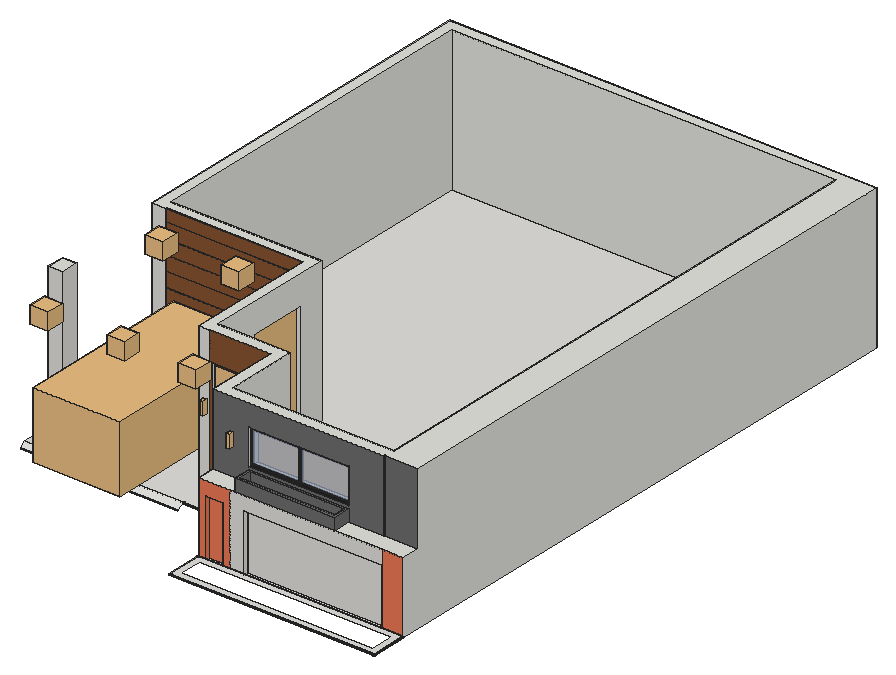
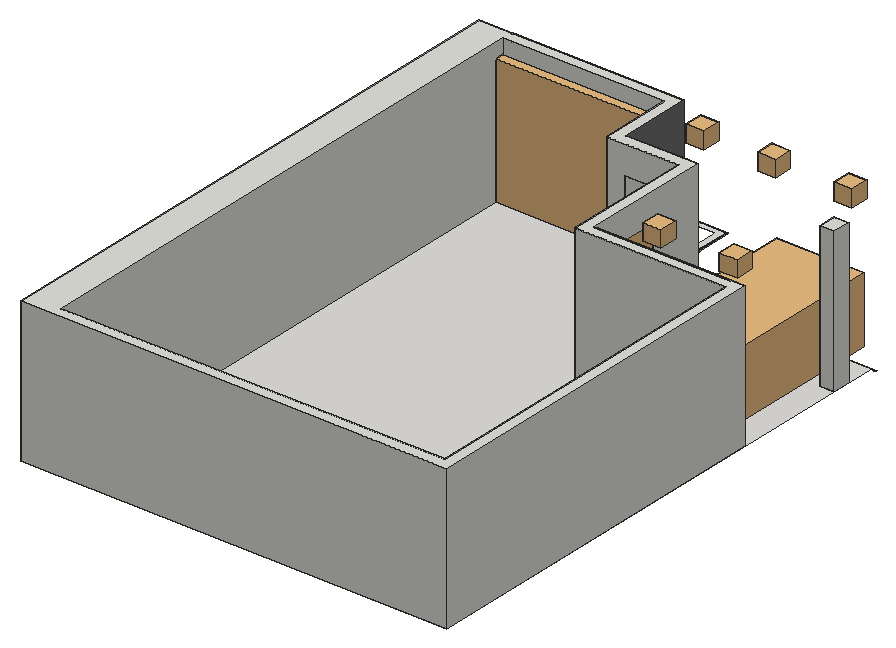
# SketchUp Ruby script. Lengths in inches.
U = 1.inch
M = Sketchup.active_model
def pt(a) = Geom::Point3d.new(a.map { |v| v * U })
def face(e, loops, mat)
  f = e.add_face(loops[0].map { |a| pt(a) })
  loops[1..].each { |l| e.add_face(l.map { |a| pt(a) }).erase! }
  f.material = f.back_material = mat if mat
  f
end
# faces: each face lists its corners as indices into pts; further lists are holes
def faces(e, pts, list, mat = nil) = list.each { |f| face(e, (f[0].is_a?(Array) ? f : [f]).map { |l| l.map { |i| pts[i] } }, mat) }
# xy, xz, yz: faces in a plane at the given z, y or x. An outline is a flat list of corners, or four numbers for a rectangle; further outlines are holes
def ring(l) = l.size == 4 ? [[l[0], l[1]], [l[2], l[1]], [l[2], l[3]], [l[0], l[3]]] : l.each_slice(2).to_a
def flat(e, list, mat, &to3) = list.each { |f| face(e, (f[0].is_a?(Array) ? f : [f]).map { |l| ring(l).map { |u, v| to3.(u, v) } }, mat) }
def xy(e, z, list, mat = nil) = flat(e, list, mat) { |x, y| [x, y, z] }
def xz(e, y, list, mat = nil) = flat(e, list, mat) { |x, z| [x, y, z] }
def yz(e, x, list, mat = nil) = flat(e, list, mat) { |y, z| [x, y, z] }
def lines(e, pts, list) = list.each { |a, b| e.add_line(pt(pts[a]), pt(pts[b])) }
# prism: a flat outline (further loops are holes) pulled along v
def prism(e, loops, v, mat = nil)
  f = face(e, loops, mat); d = Geom::Vector3d.new(v.map { |x| x * U })
  f.pushpull(f.normal.samedirection?(d) ? d.length : -d.length)
end
def box(e, o, s, mat = nil) = prism(e, [[o, [o[0] + s[0], o[1], o[2]], [o[0] + s[0], o[1] + s[1], o[2]], [o[0], o[1] + s[1], o[2]]]], [0, 0, s[2]], mat)
def at(x, y, z, deg = 0) = Geom::Transformation.translation(pt([x, y, z])) * Geom::Transformation.rotation(ORIGIN, Z_AXIS, deg.degrees)
def axes(o, x, y, z) = Geom::Transformation.new([*x, 0, *y, 0, *z, 0, *pt(o).to_a, 1])
def part(name) = M.definitions.add(name)
# library, detail: a bought-in or finely detailed component or shape, given as its bounding box
def library(name, o, s) = part(name).tap { |d| box(d.entities, o, s) }
def detail(e, o, s) = box(e.add_group.entities, o, s)
def put(e, d, t, mat = nil) = e.add_instance(d, t).tap { |i| i.material = mat if mat }
def group(e, t, mat = nil) = e.add_group.tap { |g| g.transformation = t; g.material = mat if mat }.entities
root = M.entities
M.materials.add("Wall Light").color = [248, 213, 137]
M.materials.add("[0136_Charcoal]").color = [35, 35, 35]
M.materials.add("[Formica Beige]").color = [235, 120, 86]
M.materials.add("[Formica Graystone]").color = [224, 223, 219]
M.materials.add("[Metal Rusted]").color = [135, 86, 63]
M.materials.add("[Stone Flagstone Ashlar]").color = [109, 109, 109]
M.materials.add("[Translucent Glass Blue]").color = [177, 191, 215]
M.materials["[Translucent Glass Blue]"].alpha = 0.5
M.materials.add("[Translucent Glass Blue]1").color = [190, 201, 222]
M.materials["[Translucent Glass Blue]1"].alpha = 0.5
M.materials.add("[Wood Cherry Original]").color = [134, 83, 48]
M.materials.add("[Wood Veneer 01]").color = [96, 60, 36]
c1 = library("Group\#60",[0,0,0],[55.78,24.12,15.21])
c2 = library("Flush door",[0,0,0],[29.53,2.68,82.68])
c3 = library("Component_63",[0,-41.05,1.35],[7.23,156.73,136.43])
c4 = part("1")
prism(c4.entities,[[[39.75,0,0],[0,0,0],[0,0,27],[39.75,0,27]],[[0.5,0,0.5],[39.25,0,0.5],[39.25,0,26.5],[0.5,0,26.5]]],[0,-1,0])
g1 = group(c4.entities,at(0.5,-0.75,0.5),"[Translucent Glass Blue]")
box(g1,[0,0,0],[38.75,0.47,26])
c5 = part("Group5\#1")
box(c5.entities,[-48,-60,0],[96,12,1])
c6 = part("Group6\#1")
box(c6.entities,[-48,-47.75,0],[96,12,1])
c7 = part("Group7\#1")
box(c7.entities,[-48,-35.5,0],[96,12,1])
c8 = part("Group8\#1")
box(c8.entities,[-48,-23.25,0],[96,12,1])
c9 = part("Group9\#1")
box(c9.entities,[-48,-11,0],[96,12,1])
c10 = part("Group10\#1")
box(c10.entities,[-48,1.25,0],[96,12,1])
c11 = part("Group11\#1")
box(c11.entities,[-48,13.5,0],[96,12,1])
c12 = part("Group12\#1")
box(c12.entities,[-48,25.75,0],[96,12,1])
c13 = part("Group13\#1")
box(c13.entities,[-48,38,0],[96,12,1])
c14 = part("Group14\#1")
box(c14.entities,[-48,50.25,0],[96,9.75,1])
c15 = part("Group3\#1")
put(c15.entities,c5,at(0,0,0))
put(c15.entities,c6,at(0,0,0))
put(c15.entities,c7,at(0,0,0))
put(c15.entities,c8,at(0,0,0))
put(c15.entities,c9,at(0,0,0))
put(c15.entities,c10,at(0,0,0))
put(c15.entities,c11,at(0,0,0))
put(c15.entities,c12,at(0,0,0))
put(c15.entities,c13,at(0,0,0))
put(c15.entities,c14,at(0,0,0))
c16 = library("Lattice screen panel",[0,0,-3],[165.74,168.8125,3])
c17 = part("Decorative lattice screen")
put(c17.entities,c16,at(0,0,3))
put(c17.entities,c16,axes([0,675.25,3],[1,0,0],[0,-1,0],[0,0,1]))
put(c17.entities,c16,axes([331.47,0,3],[-1,0,0],[0,1,0],[0,0,1]))
put(c17.entities,c16,at(331.47,675.25,3,180))
put(c17.entities,c16,at(331.47,337.625,3,180))
put(c17.entities,c16,at(0,337.625,3))
put(c17.entities,c16,axes([331.47,337.625,3],[-1,0,0],[0,1,0],[0,0,1]))
put(c17.entities,c16,axes([0,337.625,3],[1,0,0],[0,-1,0],[0,0,1]))
c18 = part("Jali")
put(c18.entities,c17,at(55.22,75.56,-3),"[Metal Rusted]")
g2 = group(c18.entities,at(46.22,66.56,-6))
prism(g2,[[[0,0,0],[0,693.25,0],[349.47,693.25,0],[349.47,0,0]],[[340.47,9,0],[340.47,684.25,0],[9,684.25,0],[9,9,0]]],[0,0,9])
g3 = group(c18.entities,at(46.22,66.56,-15))
g4 = group(g3,at(0,0,0))
prism(g4,[[[0,0,0],[0,693.25,0],[349.47,693.25,0],[349.47,0,0]],[[340.47,9,0],[340.47,684.25,0],[9,684.25,0],[9,9,0]]],[0,0,9])
g5 = group(g3,at(9,9,2.08))
box(g5,[0,0,0],[331.47,675.25,3.9375],"[Translucent Glass Blue]1")
c19 = library("WALL LIGHT 69",[4.19,4.05,-8.78],[4.61,5.7,17.13])
c20 = library("9",[-5.85,-5.85,-13.96],[15.28,15.28,13.96])
xy(root,25.984,[[9,195.902,141,196.152]],"[Formica Graystone]")
xy(root,29.819,[[195,150,366,150,366,645,9,645,9,201,195,201]],"[Formica Graystone]")
xy(root,30.819,[[[195,120,366,150],[200,125,361,145]]],"[Formica Graystone]")
xz(root,150,[[195,29.819,194.961,29.821,194.922,29.826,194.883,29.833,194.845,29.844,194.809,29.857,194.773,29.874,194.739,29.893,194.706,29.915,194.675,29.939,194.646,29.966,194.62,29.995,194.595,30.025,194.574,30.058,194.554,30.092,194.538,30.128,194.524,30.165,194.514,30.203,194.506,30.241,194.502,30.28,194.5,30.319,194.502,30.359,194.506,30.398,194.514,30.436,194.524,30.474,194.538,30.511,194.554,30.546,194.574,30.581,194.595,30.613,194.62,30.644,194.646,30.673,194.675,30.7,194.706,30.724,194.739,30.746,194.773,30.765,194.809,30.781,194.845,30.795,194.883,30.806,194.922,30.813,194.961,30.818,195,30.819],[195,29.819,366,30.819],[366,29.819,366,30.819,366.039,30.818,366.078,30.813,366.117,30.806,366.155,30.795,366.191,30.781,366.227,30.765,366.261,30.746,366.294,30.724,366.325,30.7,366.354,30.673,366.38,30.644,366.405,30.613,366.426,30.581,366.446,30.546,366.462,30.511,366.476,30.474,366.486,30.436,366.494,30.398,366.498,30.359,366.5,30.319,366.498,30.28,366.494,30.241,366.486,30.203,366.476,30.165,366.462,30.128,366.446,30.092,366.426,30.058,366.405,30.025,366.38,29.995,366.354,29.966,366.325,29.939,366.294,29.915,366.261,29.893,366.227,29.874,366.191,29.857,366.155,29.844,366.117,29.833,366.078,29.826,366.039,29.821]],"[Formica Graystone]")
xz(root,195.902,[[9,25.984,141,26.102]],"[Formica Graystone]")
xz(root,196.152,[[9,25.984,141,26.284]],"[Formica Graystone]")
xz(root,201,[[141,28.819,195,29.819]],"[Formica Graystone]")
yz(root,141,[[201,28.819,200.948,28.822,200.896,28.83,200.845,28.844,200.797,28.863,200.75,28.886,200.706,28.915,200.665,28.948,200.628,28.985,200.595,29.025,200.567,29.069,200.543,29.116,200.524,29.165,200.511,29.215,200.503,29.267,200.5,29.319,200.503,29.372,200.511,29.423,200.524,29.472,201,29.819],[200.524,29.472,200.524,29.474,200.543,29.523,200.567,29.569,200.595,29.613,200.628,29.654,200.665,29.691,200.706,29.724,200.75,29.752,200.797,29.776,200.845,29.795,200.896,29.808,200.948,29.817,201,29.819]],"[Formica Graystone]")
yz(root,195,[[201,28.819,200.948,28.822,200.896,28.83,200.845,28.844,200.797,28.863,200.75,28.886,200.706,28.915,200.665,28.948,200.628,28.985,200.595,29.025,200.567,29.069,200.543,29.116,200.524,29.165,200.511,29.215,200.503,29.267,200.5,29.319,200.503,29.372,200.511,29.423,200.524,29.474,200.543,29.523,200.567,29.569,200.595,29.613,200.628,29.654,200.665,29.691,200.706,29.724,200.75,29.752,200.797,29.776,200.845,29.795,200.896,29.808,200.948,29.817,201,29.819]],"[Formica Graystone]")
p = [[9,196.152,26.284],[141,196.152,26.284],[141,200.524,29.472],[141,201,29.819],[9,201,29.819],[195,200.896,28.83],
  [195,200.845,28.844],[141,200.845,28.844],[141,200.896,28.83],[195,200.797,28.863],[141,200.797,28.863],[195,201,28.819],
  [195,200.948,28.822],[141,200.948,28.822],[141,201,28.819],[195,200.665,28.948],[195,200.628,28.985],[141,200.628,28.985],
  [141,200.665,28.948],[195,200.75,28.886],[195,200.706,28.915],[141,200.706,28.915],[141,200.75,28.886],[195,200.595,29.025],
  [141,200.595,29.025],[195,200.567,29.069],[141,200.567,29.069],[195,200.543,29.116],[141,200.543,29.116],[195,200.524,29.165],
  [141,200.524,29.165],[195,200.511,29.215],[141,200.511,29.215],[195,200.503,29.267],[141,200.503,29.267],[195,200.5,29.319],
  [141,200.5,29.319],[195,200.503,29.372],[141,200.503,29.372],[195,200.511,29.423],[141,200.511,29.423],[195,200.524,29.474],
  [141,200.524,29.474],[195,200.543,29.523],[141,200.543,29.523],[195,200.567,29.569],[141,200.567,29.569],[195,200.595,29.613],
  [141,200.595,29.613],[195,200.628,29.654],[141,200.628,29.654],[195,200.665,29.691],[141,200.665,29.691],[195,200.706,29.724],
  [141,200.706,29.724],[195,200.75,29.752],[141,200.75,29.752],[194.845,150,29.844],[194.883,150,29.833],[194.883,119.883,29.833],
  [194.845,119.845,29.844],[366.117,119.883,29.833],[366.155,119.845,29.844],[194.809,150,29.857],[194.809,119.809,29.857],[366.191,119.809,29.857],
  [366.117,150,29.833],[366.155,150,29.844],[366.191,150,29.857],[194.922,150,29.826],[194.961,150,29.821],[194.961,119.961,29.821],
  [194.922,119.922,29.826],[366.039,119.961,29.821],[366.078,119.922,29.826],[366.039,150,29.821],[366.078,150,29.826],[195,150,29.819],
  [195,120,29.819],[366,120,29.819],[366,150,29.819],[195,200.797,29.776],[141,200.797,29.776],[195,200.845,29.795],
  [141,200.845,29.795],[195,200.896,29.808],[141,200.896,29.808],[195,200.948,29.817],[141,200.948,29.817],[195,201,29.819],
  [194.646,150,29.966],[194.675,150,29.939],[194.675,119.675,29.939],[194.646,119.646,29.966],[366.325,119.675,29.939],[366.354,119.646,29.966],
  [366.325,150,29.939],[366.354,150,29.966],[194.739,150,29.893],[194.773,150,29.874],[194.773,119.773,29.874],[194.739,119.739,29.893],
  [366.227,119.773,29.874],[366.261,119.739,29.893],[194.706,150,29.915],[194.706,119.706,29.915],[366.294,119.706,29.915],[366.227,150,29.874],
  [366.261,150,29.893],[366.294,150,29.915],[194.62,150,29.995],[194.62,119.62,29.995],[366.38,119.62,29.995],[194.595,150,30.025],
  [194.595,119.595,30.025],[366.405,119.595,30.025],[194.574,150,30.058],[194.574,119.574,30.058],[366.426,119.574,30.058],[366.38,150,29.995],
  [366.405,150,30.025],[366.426,150,30.058],[194.538,150,30.128],[194.554,150,30.092],[194.554,119.554,30.092],[194.538,119.538,30.128],
  [366.446,119.554,30.092],[366.462,119.538,30.128],[194.524,150,30.165],[194.524,119.524,30.165],[366.476,119.524,30.165],[366.446,150,30.092],
  [366.462,150,30.128],[366.476,150,30.165],[194.514,150,30.203],[194.514,119.514,30.203],[366.486,119.514,30.203],[194.506,150,30.241],
  [194.506,119.506,30.241],[366.494,119.506,30.241],[194.502,150,30.28],[194.502,119.502,30.28],[366.498,119.502,30.28],[366.486,150,30.203],
  [366.494,150,30.241],[366.498,150,30.28],[194.5,150,30.319],[194.5,119.5,30.319],[366.5,119.5,30.319],[194.502,150,30.359],
  [194.502,119.502,30.359],[366.498,119.502,30.359],[366.5,150,30.319],[366.498,150,30.359],[194.506,150,30.398],[194.506,119.506,30.398],
  [366.494,119.506,30.398],[194.514,150,30.436],[194.514,119.514,30.436],[366.486,119.514,30.436],[194.524,150,30.474],[194.524,119.524,30.474],
  [366.476,119.524,30.474],[366.494,150,30.398],[366.486,150,30.436],[366.476,150,30.474],[194.538,150,30.511],[194.538,119.538,30.511],
  [366.462,119.538,30.511],[194.554,150,30.546],[194.554,119.554,30.546],[366.446,119.554,30.546],[366.462,150,30.511],[366.446,150,30.546],
  [194.574,150,30.581],[194.574,119.574,30.581],[366.426,119.574,30.581],[366.426,150,30.581],[194.595,150,30.613],[194.595,119.595,30.613],
  [366.405,119.595,30.613],[194.62,150,30.644],[194.62,119.62,30.644],[366.38,119.62,30.644],[194.646,150,30.673],[194.646,119.646,30.673],
  [366.354,119.646,30.673],[366.405,150,30.613],[366.38,150,30.644],[366.354,150,30.673],[194.675,150,30.7],[194.675,119.675,30.7],
  [366.325,119.675,30.7],[366.325,150,30.7],[194.706,150,30.724],[194.706,119.706,30.724],[366.294,119.706,30.724],[194.739,150,30.746],
  [194.739,119.739,30.746],[366.261,119.739,30.746],[194.773,150,30.765],[194.773,119.773,30.765],[366.227,119.773,30.765],[366.261,150,30.746],
  [366.227,150,30.765],[366.294,150,30.724],[194.809,150,30.781],[194.809,119.809,30.781],[366.191,119.809,30.781],[194.845,150,30.795],
  [194.845,119.845,30.795],[366.155,119.845,30.795],[194.883,150,30.806],[194.883,119.883,30.806],[366.117,119.883,30.806],[366.155,150,30.795],
  [366.117,150,30.806],[366.191,150,30.781],[194.922,150,30.813],[194.922,119.922,30.813],[366.078,119.922,30.813],[194.961,150,30.818],
  [194.961,119.961,30.818],[366.039,119.961,30.818],[366.078,150,30.813],[366.039,150,30.818],[195,150,30.819],[195,120,30.819],
  [366,120,30.819],[366,150,30.819]]
faces(root,p,[[0,1,2,3,4],[5,6,7,8],[6,9,10,7],[11,12,13,14],[12,5,8,13],[15,16,17,18],[19,20,21,22],[20,15,18,21],
  [9,19,22,10],[16,23,24,17],[23,25,26,24],[25,27,28,26],[27,29,30,28],[29,31,32,30],[31,33,34,32],[33,35,36,34],
  [35,37,38,36],[37,39,40,38],[39,41,42,2,40],[41,43,44,42],[43,45,46,44],[45,47,48,46],[47,49,50,48],[49,51,52,50],
  [51,53,54,52],[53,55,56,54],[57,58,59,60],[60,59,61,62],[63,57,60,64],[64,60,62,65],[62,61,66,67],[65,62,67,68],
  [69,70,71,72],[72,71,73,74],[58,69,72,59],[59,72,74,61],[74,73,75,76],[61,74,76,66],[70,77,78,71],[71,78,79,73],
  [73,79,80,75],[55,81,82,56],[81,83,84,82],[83,85,86,84],[85,87,88,86],[87,89,3,88],[90,91,92,93],[93,92,94,95],
  [95,94,96,97],[98,99,100,101],[101,100,102,103],[104,98,101,105],[105,101,103,106],[91,104,105,92],[92,105,106,94],[103,102,107,108],
  [106,103,108,109],[94,106,109,96],[99,63,64,100],[100,64,65,102],[102,65,68,107],[110,90,93,111],[111,93,95,112],[113,110,111,114],
  [114,111,112,115],[116,113,114,117],[117,114,115,118],[112,95,97,119],[115,112,119,120],[118,115,120,121],[122,123,124,125],[125,124,126,127],
  [128,122,125,129],[129,125,127,130],[127,126,131,132],[130,127,132,133],[123,116,117,124],[124,117,118,126],[126,118,121,131],[134,128,129,135],
  [135,129,130,136],[137,134,135,138],[138,135,136,139],[140,137,138,141],[141,138,139,142],[136,130,133,143],[139,136,143,144],[142,139,144,145],
  [146,140,141,147],[147,141,142,148],[149,146,147,150],[150,147,148,151],[148,142,145,152],[151,148,152,153],[154,149,150,155],[155,150,151,156],
  [157,154,155,158],[158,155,156,159],[160,157,158,161],[161,158,159,162],[156,151,153,163],[159,156,163,164],[162,159,164,165],[166,160,161,167],
  [167,161,162,168],[169,166,167,170],[170,167,168,171],[171,168,172,173],[168,162,165,172],[174,169,170,175],[175,170,171,176],[176,171,173,177],
  [178,174,175,179],[179,175,176,180],[181,178,179,182],[182,179,180,183],[184,181,182,185],[185,182,183,186],[180,176,177,187],[183,180,187,188],
  [186,183,188,189],[190,184,185,191],[191,185,186,192],[192,186,189,193],[194,190,191,195],[195,191,192,196],[197,194,195,198],[198,195,196,199],
  [200,197,198,201],[201,198,199,202],[202,199,203,204],[196,192,193,205],[199,196,205,203],[206,200,201,207],[207,201,202,208],[209,206,207,210],
  [210,207,208,211],[212,209,210,213],[213,210,211,214],[214,211,215,216],[208,202,204,217],[211,208,217,215],[218,212,213,219],[219,213,214,220],
  [221,218,219,222],[222,219,220,223],[223,220,224,225],[220,214,216,224],[226,221,222,227],[227,222,223,228],[228,223,225,229]],"[Formica Graystone]")
put(root,c1,axes([30.83,328.8125,29.82],[0,-2.64,0],[3.036,0,0],[0,0,3.67488]))
g6 = group(root,at(9,150,29.82))
xy(g6,0,[[186,0,186,75,180,75,180,84,195,84,195,24,330,24,330,486,9,486,9,192,135,192,135,171,126,171,126,184,12,184,12,183,0,183,0,495,357,495,357,0,339,0,339,3,339.5,3,339.5,4,223.5,4,223.5,3,224,3,224,0,206,0,206,3,206.5,3,206.5,4,191.5,4,191.5,3,192,3,192,0],[0,75,12,90],[126,75,126,121,135,121,135,84,138,84,138,75],[138,78,180,84]])
xy(g6,0.15,[[191.65,2.75,191.85,3],[206.15,2.75,206.35,3]])
xy(g6,0.16,[[223.66,2.75,223.84,3],[339.16,2.75,339.34,3]])
xy(g6,48,[[192,0,206,3]],"[Formica Beige]")
xy(g6,48,[[224,0,339,3]],"[Formica Graystone]")
xy(g6,48.15,[[191.85,2.75,206.15,3]])
xy(g6,48.16,[[223.84,2.75,339.16,3]])
xy(g6,48.34,[[223.66,2.75,339.34,3]])
xy(g6,48.35,[[191.65,2.75,206.35,3]])
xy(g6,48.5,[[223.5,3,339.5,4]])
xy(g6,48.5,[[191.5,3,206.5,4]],"[Formica Beige]")
xy(g6,60,[[186,0,357,0,357,15,330,15,330,15.5,329,15.5,329,15,186,15]])
xy(g6,72,[[216,15,300,24]])
xy(g6,96,[[138,75,180,78],[138,78,180,84]])
xy(g6,96,[[126,121,135,171]],"[Formica Graystone]")
xy(g6,102,[[216,15,300,24]])
xy(g6,120,[[[186,15,329,15,329,15.5,330,15.5,330,15,357,15,357,495,0,495,0,183,12,183,12,184,126,184,126,75,186,75],[195,24,195,84,135,84,135,192,9,192,9,486,330,486,330,24]],[0,75,12,90]])
xz(g6,0,[[186,0,192,0,192,48,206,48,206,0,212,0,212,60,186,60],[339,0,357,60]],"[Formica Beige]")
xz(g6,0,[[212,0,224,0,224,48,339,48,339,60,212,60]],"[Formica Graystone]")
xz(g6,2.75,[[191.65,0.15,191.65,48.35,206.35,48.35,206.35,0.15,206.15,0.15,206.15,48.15,191.85,48.15,191.85,0.15],[223.66,0.16,223.66,48.34,339.34,48.34,339.34,0.16,339.16,0.16,339.16,48.16,223.84,48.16,223.84,0.16]])
xz(g6,3,[[[191.5,0,191.5,48.5,206.5,48.5,206.5,0,206,0,206,48,192,48,192,0],[191.65,0.15,191.85,0.15,191.85,48.15,206.15,48.15,206.15,0.15,206.35,0.15,206.35,48.35,191.65,48.35]],[[223.5,0,223.5,48.5,339.5,48.5,339.5,0,339,0,339,48,224,48,224,0],[223.66,0.16,223.84,0.16,223.84,48.16,339.16,48.16,339.16,0.16,339.34,0.16,339.34,48.34,223.66,48.34]]])
xz(g6,4,[[191.5,0,206.5,48.5]],"[Formica Beige]")
xz(g6,4,[[223.5,0,339.5,48.5]],"[Formica Graystone]")
xz(g6,15,[[[186,60,329,120],[216,72,300,102]],[330,60,357,120]],"[Stone Flagstone Ashlar]")
xz(g6,15.5,[[329,60,330,120]])
xz(g6,24,[[[195,0,330,120],[216,72,300,102]]])
xz(g6,75,[[0,0,12,120],[126,0,135,120]],"[Formica Graystone]")
xz(g6,75,[[135,0,138,0,138,96,180,96,180,0,186,0,186,120,135,120]],"[Wood Cherry Original]")
xz(g6,78,[[138,0,180,96]])
xz(g6,84,[[135,0,135,120,195,120,195,0,180,0,180,96,138,96,138,0],[138,0,180,96]])
xz(g6,90,[[0,0,12,120]])
xz(g6,121,[[126,0,135,96]])
xz(g6,171,[[126,0,135,96]],"[Formica Graystone]")
xz(g6,183,[[0,0,12,120]],"[Formica Graystone]")
xz(g6,184,[[12,0,126,120]])
xz(g6,192,[[9,0,135,120]])
xz(g6,486,[[9,0,330,120]])
xz(g6,495,[[0,0,357,120]])
yz(g6,0,[[75,0,90,120],[183,0,495,120]],"[Formica Graystone]")
yz(g6,9,[[192,0,486,120]])
yz(g6,12,[[183,0,184,120]])
yz(g6,12,[[75,0,90,120]],"[Formica Graystone]")
yz(g6,126,[[75,0,75,120,184,120,184,0,171,0,171,96,121,96,121,0]],"[Formica Graystone]")
yz(g6,135,[[84,0,121,0,121,96,171,96,171,0,192,0,192,120,84,120]])
yz(g6,138,[[75,0,78,96],[78,0,84,96]])
yz(g6,180,[[75,0,78,96],[78,0,84,96]])
yz(g6,186,[[0,0,0,60,15,60,15,120,75,120,75,0]],"[Stone Flagstone Ashlar]")
yz(g6,191.5,[[3,0,4,48.5]],"[Formica Beige]")
yz(g6,191.65,[[2.75,0.15,3,48.35]])
yz(g6,191.85,[[2.75,0.15,3,48.15]])
yz(g6,192,[[0,0,3,48]],"[Formica Beige]")
yz(g6,195,[[24,0,84,120]])
yz(g6,206,[[0,0,3,48]],"[Formica Beige]")
yz(g6,206.15,[[2.75,0.15,3,48.15]])
yz(g6,206.35,[[2.75,0.15,3,48.35]])
yz(g6,206.5,[[3,0,4,48.5]],"[Formica Beige]")
yz(g6,216,[[15,72,24,102]])
yz(g6,223.5,[[3,0,4,48.5]])
yz(g6,223.66,[[2.75,0.16,3,48.34]])
yz(g6,223.84,[[2.75,0.16,3,48.16]])
yz(g6,224,[[0,0,3,48]],"[Formica Graystone]")
yz(g6,300,[[15,72,24,102]])
yz(g6,329,[[15,60,15.5,120]])
yz(g6,330,[[24,0,486,120],[15,60,15.5,120]])
yz(g6,339,[[0,0,3,48]],"[Formica Graystone]")
yz(g6,339.16,[[2.75,0.16,3,48.16]])
yz(g6,339.34,[[2.75,0.16,3,48.34]])
yz(g6,339.5,[[3,0,4,48.5]])
yz(g6,357,[[0,0,495,0,495,120,15,120,15,60,0,60]])
put(g6,c2,axes([130.68,121,0],[0,1.69333,0],[-1,0,0],[0,0,1.16114]))
put(g6,c3,axes([294.64,24,108.85],[0,1,0],[-0.86133,0,0],[0,0,-0.79]))
g7 = group(g6,at(216,18,72),"[0136_Charcoal]")
prism(g7,[[[0,0,0],[0,0,30],[84,0,30],[84,0,0]],[[41.25,0,1.5],[41.25,0,28.5],[1.5,0,28.5],[1.5,0,1.5]],[[42.75,0,1.5],[82.5,0,1.5],[82.5,0,28.5],[42.75,0,28.5]]],[0,-2,0])
put(g7,c4,at(1.5,-0.5,1.5))
put(g7,c4,at(42.75,-0.5,1.5))
g8 = group(g6,at(12,184,0))
put(g8,c15,axes([57,0,60],[1.1875,0,0],[0,0,1],[0,-1,0]),"[Wood Cherry Original]")
g9 = group(g6,at(216,0,60),"[Stone Flagstone Ashlar]")
xy(g9,0,[[0,0,84,15]])
xy(g9,1,[[2.5,2.5,81.5,12.5]])
xy(g9,10,[[[0,0,84,15],[2.5,2.5,81.5,12.5]]])
xz(g9,0,[[0,0,84,10]])
xz(g9,2.5,[[2.5,1,81.5,10]])
xz(g9,12.5,[[2.5,1,81.5,10]])
xz(g9,15,[[0,0,84,10]])
yz(g9,0,[[0,0,15,10]])
yz(g9,2.5,[[2.5,1,12.5,10]])
yz(g9,81.5,[[2.5,1,12.5,10]])
yz(g9,84,[[0,0,15,10]])
g10 = group(g6,at(329,15.5,60),"Wall Light")
box(g10,[0,-0.5,0],[1,0.5,60])
g11 = group(g6,at(191.65,2.75,0.15),"Wall Light")
prism(g11,[[[14.5,0,0],[14.7,0,0],[14.7,0,48.2],[0,0,48.2],[0,0,0],[0.2,0,0],[0.2,0,48],[14.5,0,48]]],[0,0.25,0])
g12 = group(g6,at(223.66,2.75,0.16),"Wall Light")
prism(g12,[[[0.18,0,0],[0.18,0,48],[115.5,0,48],[115.5,0,0],[115.68,0,0],[115.68,0,48.18],[0,0,48.18],[0,0,0]]],[0,0.25,0])
put(root,c18,axes([141.45,225.86,20.6],[0.12,0,0],[0,0,0.13848],[0,-0.12,0]),"[Wood Veneer 01]")
put(root,c19,axes([135.875,218.66,91.3],[0.65,0,0],[0,0.65,0],[0,0,0.65]))
put(root,c19,axes([206.21,158.66,117.65],[0.65,0,0],[0,0.65,0],[0,0,0.65]))
put(root,c20,at(103.21,181.28,151.07))
put(root,c20,at(163.16,181.28,151.07))
put(root,c20,at(103.16,301.28,151.07))
put(root,c20,at(39.28,181.21,151.07))
put(root,c20,at(39.28,301.21,151.07))
